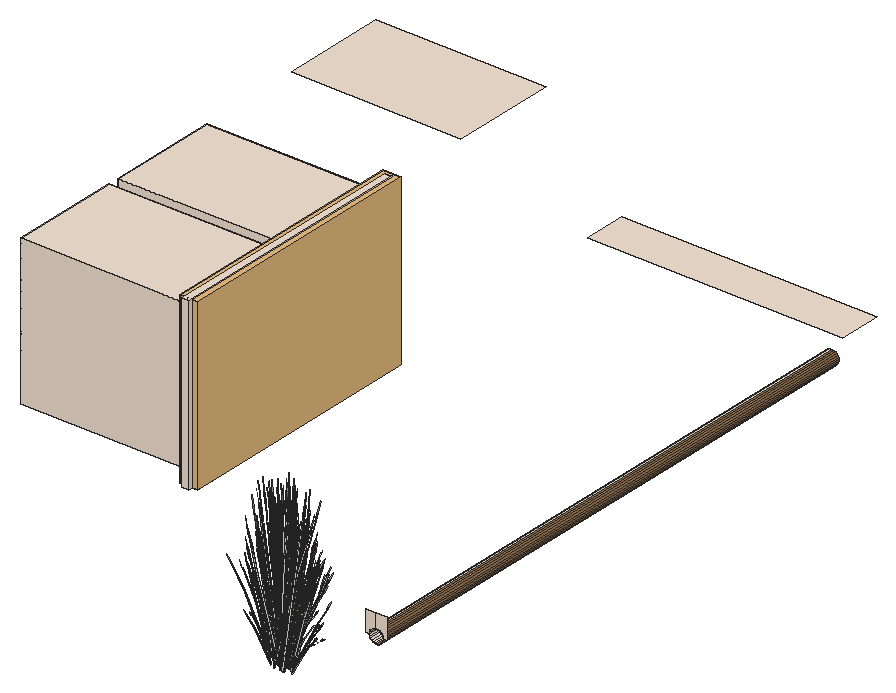
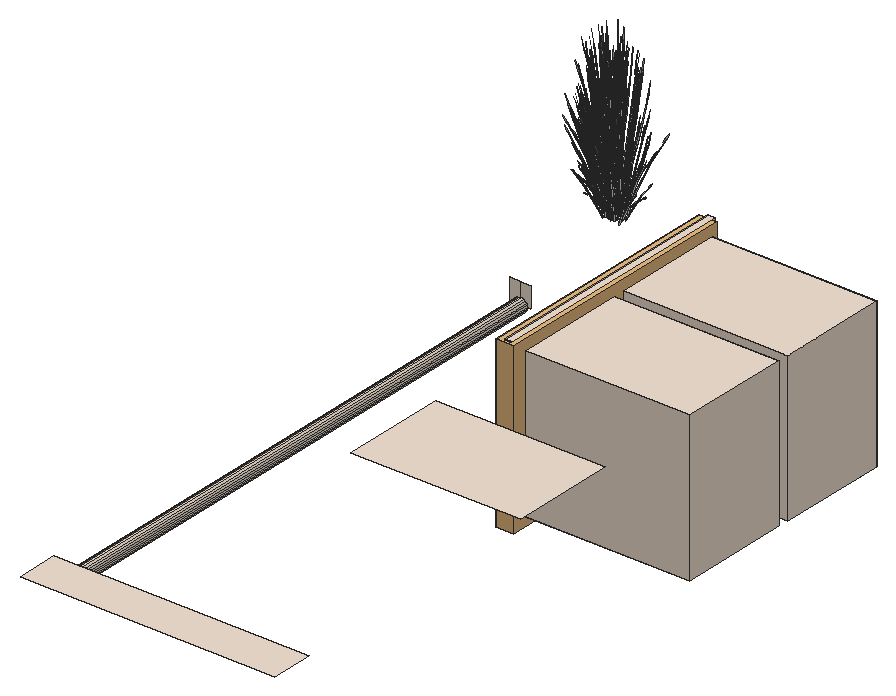
# SketchUp Ruby script. Lengths in inches.
U = 1.inch
M = Sketchup.active_model
def pt(a) = Geom::Point3d.new(a.map { |v| v * U })
def face(e, loops, mat)
  f = e.add_face(loops[0].map { |a| pt(a) })
  loops[1..].each { |l| e.add_face(l.map { |a| pt(a) }).erase! }
  f.material = f.back_material = mat if mat
  f
end
# faces: each face lists its corners as indices into pts; further lists are holes
def faces(e, pts, list, mat = nil) = list.each { |f| face(e, (f[0].is_a?(Array) ? f : [f]).map { |l| l.map { |i| pts[i] } }, mat) }
# xy, xz, yz: faces in a plane at the given z, y or x. An outline is a flat list of corners, or four numbers for a rectangle; further outlines are holes
def ring(l) = l.size == 4 ? [[l[0], l[1]], [l[2], l[1]], [l[2], l[3]], [l[0], l[3]]] : l.each_slice(2).to_a
def flat(e, list, mat, &to3) = list.each { |f| face(e, (f[0].is_a?(Array) ? f : [f]).map { |l| ring(l).map { |u, v| to3.(u, v) } }, mat) }
def xy(e, z, list, mat = nil) = flat(e, list, mat) { |x, y| [x, y, z] }
def xz(e, y, list, mat = nil) = flat(e, list, mat) { |x, z| [x, y, z] }
def yz(e, x, list, mat = nil) = flat(e, list, mat) { |y, z| [x, y, z] }
def lines(e, pts, list) = list.each { |a, b| e.add_line(pt(pts[a]), pt(pts[b])) }
# prism: a flat outline (further loops are holes) pulled along v
def prism(e, loops, v, mat = nil)
  f = face(e, loops, mat); d = Geom::Vector3d.new(v.map { |x| x * U })
  f.pushpull(f.normal.samedirection?(d) ? d.length : -d.length)
end
def box(e, o, s, mat = nil) = prism(e, [[o, [o[0] + s[0], o[1], o[2]], [o[0] + s[0], o[1] + s[1], o[2]], [o[0], o[1] + s[1], o[2]]]], [0, 0, s[2]], mat)
def at(x, y, z, deg = 0) = Geom::Transformation.translation(pt([x, y, z])) * Geom::Transformation.rotation(ORIGIN, Z_AXIS, deg.degrees)
def axes(o, x, y, z) = Geom::Transformation.new([*x, 0, *y, 0, *z, 0, *pt(o).to_a, 1])
def part(name) = M.definitions.add(name)
# library, detail: a bought-in or finely detailed component or shape, given as its bounding box
def library(name, o, s) = part(name).tap { |d| box(d.entities, o, s) }
def detail(e, o, s) = box(e.add_group.entities, o, s)
def put(e, d, t, mat = nil) = e.add_instance(d, t).tap { |i| i.material = mat if mat }
def group(e, t, mat = nil) = e.add_group.tap { |g| g.transformation = t; g.material = mat if mat }.entities
root = M.entities
M.materials.add("C01_Vanilla_Cream").color = [244, 228, 212]
M.materials.add("LightPink_Translucent").color = [144, 107, 117]
M.materials["LightPink_Translucent"].alpha = 0.75
M.materials.add("Wood_Floor_01_1K").color = [146, 111, 76]
c1 = part("blade")
p = [[2.15,0.21,22],[0,0.17,0],[0.09,0.45,0],[2.18,0.31,22],[2.29,0.31,22],[0.38,0.45,0],
  [2.48,0.24,33],[2.49,0.24,33],[2.48,0.22,33]]
faces(c1.entities,p,[[0,1,2,3],[4,5,2,3],[6,3,4,7],[8,0,3,6]])
c2 = part("seeds")
p = [[0.3,-0.1,1.38],[-0.01,-0.03,1.59],[-0.01,-0.03,0.03],[0.14,-0.07,-0.07],[0.29,-0.03,3],[0.15,0.01,3.11]]
faces(c2.entities,p,[[0,1,2,3],[1,0,4,5]],"LightPink_Translucent")
c3 = part("blade with seeds")
put(c3.entities,c1,at(0,0,0))
put(c3.entities,c2,axes([2.4,0.25,30.99],[1.5799,-0.05474,1.17369],[-0.12525,1.92788,0.29478],[-0.07173,-0.02425,1.56792]))
c4 = library("Double casement window",[0,0,0],[5.02,56.42,60])
xy(root,198,[[288,324,290,396],[288,468,360,480]],"C01_Vanilla_Cream")
xy(root,201,[[240,327,290,358.5],[240,361.5,290,393]],"C01_Vanilla_Cream")
xy(root,243,[[240,327,290,358.5],[240,361.5,290,393],[240,423,288,453]],"C01_Vanilla_Cream")
xy(root,246,[[288,324,290,396]],"C01_Vanilla_Cream")
xz(root,306.76,[[354,192,354,198,357,198,357,194,356.48,193.93,356,193.73,355.59,193.41,355.27,193,355.07,192.52,355,192],[359,192,358.93,192.52,358.73,193,358.41,193.41,358,193.73,357.52,193.93,357,194,357,198,360,198,360,192]],"C01_Vanilla_Cream")
xz(root,324,[[288,198,290,246]],"C01_Vanilla_Cream")
xz(root,327,[[240,201,290,243]],"C01_Vanilla_Cream")
xz(root,358.5,[[240,201,290,243]],"C01_Vanilla_Cream")
xz(root,361.5,[[240,201,290,243]],"C01_Vanilla_Cream")
xz(root,393,[[240,201,290,243]],"C01_Vanilla_Cream")
xz(root,396,[[288,198,290,246]],"C01_Vanilla_Cream")
yz(root,240,[[327,201,358.5,243],[361.5,201,393,243]],"C01_Vanilla_Cream")
yz(root,290,[[[324,198,396,246],[327,201,358.5,243],[361.5,201,393,243]]],"C01_Vanilla_Cream")
p = [[357,306.76,190],[356.48,306.76,190.07],[356.48,468,190.07],[357,468,190],[357.52,306.76,190.07],[357.52,468,190.07],
  [356,306.76,190.27],[356,468,190.27],[358,306.76,190.27],[358,468,190.27],[355.59,306.76,190.59],[355.59,468,190.59],
  [358.41,306.76,190.59],[358.41,468,190.59],[355.27,306.76,191],[355.27,468,191],[358.73,306.76,191],[358.73,468,191],
  [355.07,306.76,191.48],[355.07,468,191.48],[358.93,306.76,191.48],[358.93,468,191.48],[355,306.76,192],[355,468,192],
  [359,306.76,192],[359,468,192],[355.07,306.76,192.52],[355.07,468,192.52],[358.93,306.76,192.52],[358.93,468,192.52],
  [355.27,306.76,193],[355.27,468,193],[358.73,306.76,193],[358.73,468,193],[355.59,306.76,193.41],[355.59,468,193.41],
  [358.41,306.76,193.41],[358.41,468,193.41],[356,306.76,193.73],[356,468,193.73],[358,306.76,193.73],[358,468,193.73],
  [356.48,306.76,193.93],[356.48,468,193.93],[357.52,306.76,193.93],[357.52,468,193.93],[357,306.76,194],[357,468,194]]
faces(root,p,[[0,1,2,3],[1,6,7,2],[6,10,11,7],[10,14,15,11],[14,18,19,15],[18,22,23,19],[22,26,27,23],[26,30,31,27],
  [30,34,35,31],[34,38,39,35],[38,42,43,39],[42,46,47,43]],"C01_Vanilla_Cream")
faces(root,p,[[4,0,3,5],[8,4,5,9],[12,8,9,13],[16,12,13,17],[20,16,17,21],[24,20,21,25],[28,24,25,29],[32,28,29,33],
  [36,32,33,37],[40,36,37,41],[44,40,41,45],[46,44,45,47]],"Wood_Floor_01_1K")
put(root,c3,axes([359.88,272.5,201.51],[0.15083,-0.44814,-0.38324],[0.51712,0.15361,-0.29685],[0.2082,-0.04109,0.7333]))
put(root,c3,axes([359.0625,270.67,199.78],[0.34808,-0.49367,0],[0.58235,0.27531,-0.38706],[0.13264,0.0627,1.22783]))
put(root,c3,axes([354.96,271.65,200.91],[0.23093,-0.01116,1.28532],[-0.15319,0.4836,0.10393],[-0.32909,-0.02991,0.54946]))
put(root,c3,axes([356.98,272.78,199.66],[-0.33445,-0.41351,-0.33554],[0.50659,-0.29119,0.16149],[-0.10823,-0.05117,1.07733]))
put(root,c3,axes([357.05,272.2,199.77],[0.24206,0.5509,0.34316],[-0.69162,0.19157,0.13466],[0.00845,-0.10123,1.19142]))
put(root,c3,axes([360.43,272.625,199.49],[-0.35858,0.05912,1.06187],[-0.05708,-0.47061,0.06078],[0.25115,-0.07123,0.60425]))
put(root,c3,axes([361.08,272.21,199.7],[-0.34516,-0.31503,-0.04866],[0.37803,-0.28865,-0.22062],[0.10711,-0.02032,0.72768]))
put(root,c3,axes([356.92,272.63,200.04],[-0.27012,0.44393,0.33554],[-0.56127,-0.21365,-0.16149],[0,-0.10233,1.07733]))
put(root,c3,axes([357.92,272.25,199.65],[0,-0.57005,0],[0.69617,0,0],[0,0,1.34592]))
put(root,c3,axes([358.76,270.93,199.86],[-0.52105,-0.24633,0.37238],[0.31144,-0.44171,0],[0.11867,0.0561,1.18128]))
put(root,c3,axes([359.78,272.66,201.74],[0.48922,-0.21758,-0.53284],[0.27264,0.44789,0.0643],[0.23638,-0.05088,0.75375]))
put(root,c3,axes([356.68,272.94,199.54],[-0.57914,-0.08077,-0.46765],[0.12221,-0.49823,-0.12274],[-0.17283,-0.06037,1.03225]))
put(root,c3,axes([357.59,271.89,199.77],[-0.46162,0.4471,0.34316],[-0.54842,-0.39467,0.13466],[0.11129,-0.04462,1.19142]))
put(root,c3,axes([358.09,272.6875,199.72],[-0.51786,-0.42404,-0.04598],[0.51817,-0.4243,0],[-0.01808,-0.01481,1.31678]))
put(root,c3,axes([356.79,271.15,199.86],[-0.16083,0.48962,0.13232],[-0.58854,-0.13856,0.26315],[0.10167,-0.00238,1.20305]))
put(root,c3,axes([359.71,272.75,201.79],[-0.46269,-0.13744,0.2656],[0.13495,-0.40096,-0.3429],[0.18628,-0.03677,0.65611]))
put(root,c3,axes([354.86,272.01,201.55],[0.15729,-0.44921,0.36002],[0.51712,0.15361,0.29685],[-0.20336,0.027,0.74497]))
put(root,c3,axes([356.54,271.55,199.2],[-0.548,0.19724,0.96696],[-0.17442,-0.56594,0.37572],[0.3365,0.00941,1.09981]))
put(root,c3,axes([358.01,271.7,199.96],[0.1074,-0.43968,0.1086],[0.52474,0.07632,-0.3101],[0.0955,0.04515,0.95058]))
put(root,c3,axes([354.83,271.89,201.55],[-0.20448,-0.33592,0.04823],[0.37288,-0.16442,0.37966],[-0.16437,0.03244,0.57892]))
put(root,c3,axes([357.11,272.74,199.77],[0.70367,0.1038,0.34316],[-0.1432,0.58624,0.13466],[-0.10283,-0.05661,1.19142]))
put(root,c3,axes([360.82,272.32,199.12],[-0.0291,-0.0748,1.32257],[0.20181,-0.43752,-0.20205],[0.20357,-0.00629,0.22528]))
put(root,c3,axes([354.81,272.24,199.12],[0.01412,0.07764,1.32257],[-0.28464,0.40547,-0.20205],[-0.20218,-0.02044,0.22528]))
put(root,c3,axes([357.79,271.8125,200.04],[-0.33445,-0.41351,0.33554],[0.50659,-0.29119,-0.16149],[0.10823,0.05117,1.07733]))
put(root,c3,axes([356.0625,273.7,199.52],[-0.13078,-0.42928,-0.23233],[0.51941,-0.1219,0.23233],[-0.10471,-0.0495,1.0423]))
put(root,c3,axes([356.73,273.68,199.86],[0.59825,-0.13076,0.13232],[0.14773,0.48663,0.26315],[-0.05336,-0.0709,1.20305]))
put(root,c3,axes([357.96,271.84,200],[0.56211,-0.32708,-0.21822],[0.3738,0.46216,-0.37502],[0.13869,0.04694,1.19781]))
put(root,c3,axes([360.2,272.7,201.39],[0.46269,0.13744,-0.2656],[-0.13495,0.40096,0.3429],[0.18628,-0.03677,0.65611]))
put(root,c3,axes([355.92,273.89,199.51],[-0.52105,-0.24633,-0.37238],[0.31144,-0.44171,0],[-0.11867,-0.0561,1.18128]))
put(root,c3,axes([359.38,270.97,199.51],[0.52105,0.24633,-0.37238],[-0.31144,0.44171,0],[0.11867,0.0561,1.18128]))
put(root,c3,axes([354.76,272.0625,201.39],[-0.46269,-0.13744,-0.2656],[0.13495,-0.40096,0.3429],[-0.18628,0.03677,0.65611]))
put(root,c3,axes([358.39,272.375,199.65],[0.62289,0,0],[0,0.51004,0],[0,0,1.33805]))
put(root,c3,axes([357.33,273.02,200],[-0.56211,0.32708,-0.21822],[-0.3738,-0.46216,-0.37502],[-0.13869,-0.04694,1.19781]))
put(root,c3,axes([358.57,271.18,199.86],[-0.59825,0.13076,0.13232],[-0.14773,-0.48663,0.26315],[0.05336,0.0709,1.20305]))
put(root,c3,axes([358.93,272.21,200.91],[-0.23093,0.01116,1.28532],[0.15319,-0.4836,0.10393],[0.32909,0.02991,0.54946]))
put(root,c3,axes([359.23,271.15,199.52],[0.13078,0.42928,-0.23233],[-0.51941,0.1219,0.23233],[0.10471,0.0495,1.0423]))
put(root,c3,axes([360.13,272.87,201.55],[0.20448,0.33592,0.04823],[-0.37288,0.16442,0.37966],[0.16437,-0.03244,0.57892]))
put(root,c3,axes([358.1875,272.12,199.79],[-0.70367,-0.1038,0.36899],[0.1432,-0.58624,0.1448],[0.10283,0.05661,1.2811]))
put(root,c3,axes([360.09,272.75,201.55],[-0.15729,0.44921,0.36002],[-0.51712,-0.15361,0.29685],[0.20336,-0.027,0.74497]))
put(root,c3,axes([357.625,273.5625,199.65],[-0.18165,-0.42474,0],[0.51872,-0.14874,0],[0,0,1.15778]))
put(root,c3,axes([357.28,273.16,199.96],[-0.1074,0.43968,0.1086],[-0.52474,-0.07632,-0.3101],[-0.0955,-0.04515,0.95058]))
put(root,c3,axes([355.24,272.02,201.79],[0.46269,0.13744,0.2656],[-0.13495,0.40096,-0.3429],[-0.18628,0.03677,0.65611]))
put(root,c3,axes([358.31,273.5,199.64],[0.5845,-0.16716,-0.14398],[0.20539,0.48152,0.00006],[0.06452,-0.01848,1.30423]))
put(root,c3,axes([358.51,273.7,199.86],[0.16083,-0.48962,0.13232],[0.58854,0.13856,0.26315],[-0.10167,0.00238,1.20305]))
put(root,c3,axes([358.375,272.59,199.66],[0.38863,0.31822,0],[-0.38863,0.31822,0],[0,0,1.2695]))
put(root,c3,axes([356.17,272,200.51],[0.15825,-0.07127,1.32798],[0.05457,0.4976,0.10393],[-0.34278,0.06603,0.47463]))
put(root,c3,axes([359.43,272.45,199.86],[-0.43742,-0.35886,0.13232],[0.44081,-0.34807,0.26315],[-0.04831,0.07329,1.20305]))
put(root,c3,axes([358.62,271.91,199.54],[0.57914,0.08077,-0.46765],[-0.12221,0.49823,-0.12274],[0.17283,0.06037,1.03225]))
put(root,c3,axes([361.18,272.78,200.07],[-0.34399,0.08133,0.86145],[0.16192,-0.33614,0.63294],[0.18249,0.023,0.18974]))
put(root,c3,axes([357.5,273.75,199.65],[-0.56127,-0.22118,0],[0.27012,-0.45959,0],[0,0,1.2203]))
put(root,c3,axes([357.96,273.17,199.85],[-0.54364,-0.39653,-0.18894],[0.45745,-0.44527,0.41347],[-0.14639,0.04639,1.26162]))
put(root,c3,axes([356.53,273.93,199.86],[0.52105,0.24633,0.37238],[-0.31144,0.44171,0],[-0.11867,-0.0561,1.18128]))
put(root,c3,axes([358.37,272.22,200.04],[0.27012,-0.44393,0.33554],[0.56127,0.21365,-0.16149],[0,0.10233,1.07733]))
put(root,c3,axes([361.02,274.21,201.53],[-0.05034,-0.04313,1.33037],[0.11012,-0.46232,-0.12571],[0.1983,-0.02954,0.23543]))
put(root,c3,axes([354.47,272.33,201.54],[-0.09091,0.06396,1.31208],[0.00773,0.46734,-0.2075],[-0.20839,0.06078,0.10523]))
put(root,c3,axes([358.27,272.48,199.72],[0,0.56976,-0.04228],[-0.69617,0,0],[0,0.01791,1.34526]))
put(root,c3,axes([355.07,272.27,201.51],[-0.15083,0.44814,-0.38324],[-0.51712,-0.15361,-0.29685],[-0.2082,0.04109,0.7333]))
put(root,c3,axes([355.05,271.88,201.78],[0.28012,0.44611,-0.0912],[-0.49717,0.21923,-0.50621],[-0.20951,0.05886,0.76918]))
put(root,c3,axes([358.32,272.07,199.66],[0.33445,0.41351,-0.33554],[-0.50659,0.29119,0.16149],[0.10823,0.05117,1.07733]))
put(root,c3,axes([360.58,273.82,200.95],[-0.10656,-0.41414,-0.02619],[0.50364,-0.09521,-0.11874],[0.10517,0.02626,0.39164]))
put(root,c3,axes([356.23,274.18,199.78],[-0.34808,0.49367,0],[-0.58235,-0.27531,-0.38706],[-0.13264,-0.0627,1.22783]))
put(root,c3,axes([359.27,273.81,201.78],[0.02981,-0.50103,-0.0912],[0.56442,0.01369,-0.50621],[0.21738,0.0348,0.76918]))
put(root,c3,axes([359.79,272.47,199.86],[0,-0.49266,0.37238],[0.62289,0,0],[0,0.11221,1.18128]))
put(root,c3,axes([358.23,272.84,200.04],[0.60457,-0.03041,0.33554],[0.05467,0.50484,-0.16149],[-0.10823,0.05117,1.07733]))
put(root,c3,axes([358.6,272.32,199.96],[0.51872,-0.14368,0.1086],[0.18165,0.41027,-0.3101],[0,0.09029,0.95058]))
put(root,c3,axes([359.1875,273.61,201.79],[-0.31678,-0.30846,0.2656],[0.36171,-0.29199,-0.3429],[0.18378,0.04443,0.65611]))
put(root,c3,axes([357.6875,273.08,199.66],[-0.60457,0.03041,-0.33554],[-0.05467,-0.50484,0.16149],[-0.10823,0.05117,1.07733]))
put(root,c3,axes([360.53,273.32,199.94],[-0.13408,-0.12117,1.07251],[0.17446,-0.40083,-0.23066],[0.27128,0.0543,0.45856]))
put(root,c3,axes([358.14,273.76,199.65],[0.56127,0.22118,0],[-0.27012,0.45959,0],[0,0,1.31215]))
put(root,c3,axes([359.76,273.51,201.54],[0.11943,-0.00833,1.31208],[0.32759,-0.38275,-0.2075],[0.21244,0.05052,0.10523]))
put(root,c3,axes([358.36,274.25,199.64],[-0.34375,-0.4954,-0.03857],[0.58235,-0.27531,0.38706],[-0.1435,0.04717,1.22723]))
put(root,c3,axes([358.24,273.05,199.96],[0.41131,0.296,0.1086],[-0.34309,0.33395,-0.3101],[-0.0955,0.04515,0.95058]))
put(root,c3,axes([354.99,273.13,201.55],[-0.13808,-0.45342,0.36002],[0.54163,-0.07869,0.29685],[-0.15963,0.10664,0.74497]))
put(root,c3,axes([354.88,273.04,201.55],[-0.3822,-0.20719,0.04823],[0.22252,-0.29505,0.37966],[-0.12254,0.09539,0.57892]))
put(root,c3,axes([355.06,272.5,200.91],[0.19317,-0.10421,1.28532],[0.16263,0.48153,0.10393],[-0.30326,0.10883,0.54946]))
put(root,c3,axes([359.3,273.57,201.74],[0.55654,0.01186,-0.53284],[-0.03738,0.49951,0.0643],[0.23578,0.05271,0.75375]))
put(root,c3,axes([358.67,273.97,199.86],[0.52105,-0.24633,0.37238],[0.31144,0.44171,0],[-0.11867,0.0561,1.18128]))
put(root,c3,axes([357.93,273.58,199.72],[0.24206,0.56598,-0.04509],[-0.69162,0.19832,0],[0.00845,0.01976,1.2913]))
put(root,c3,axes([358.2,274.19,199.52],[-0.51941,-0.1219,-0.23233],[0.13078,-0.42928,0.23233],[-0.10471,0.0495,1.0423]))
put(root,c3,axes([354.45,273.32,199.94],[0.19348,0.04044,1.07251],[0.1247,0.41309,-0.23066],[-0.26282,0.07733,0.45856]))
put(root,c3,axes([355.32,272.98,201.79],[0.48462,-0.07041,0.2656],[0.12797,0.4025,-0.3429],[-0.13888,0.10811,0.65611]))
put(root,c3,axes([360.21,272.55,199.78],[0.69617,0,0],[0,0.55062,-0.38706],[0,0.12541,1.22783]))
put(root,c3,axes([353.46,272.8,201.53],[0.07105,0.01321,1.33037],[0.2198,0.43529,-0.12571],[-0.14545,0.11425,0.23543]))
put(root,c3,axes([359.93,272.84,199.65],[-0.69582,-0.00394,-0.03732],[0,-0.55062,0.37457],[-0.02187,0.12535,1.18764]))
put(root,c3,axes([358.43,272.36,200],[0.62699,0.23507,-0.21822],[-0.3019,0.49615,-0.37502],[0.0197,0.12182,1.19781]))
put(root,c3,axes([354.05,274.18,200.07],[0.23202,-0.22328,0.86145],[0.09155,0.35348,0.63294],[-0.16768,0.06329,0.18974]))
put(root,c3,axes([359.64,273.77,201.39],[0.31678,0.30846,-0.2656],[-0.36171,0.29199,0.3429],[0.18378,0.04443,0.65611]))
put(root,c3,axes([359.79,272.92,199.52],[-0.38863,0.30738,-0.23233],[-0.38863,-0.30738,0.23233],[0,0.09901,1.0423]))
put(root,c3,axes([358.11,272.95,200],[0.06488,0.56215,-0.21822],[-0.6757,0.03399,-0.37502],[-0.11898,0.07488,1.19781]))
put(root,c3,axes([359.47,273.89,201.55],[-0.02803,0.37463,0.04823],[-0.42332,-0.01027,0.37966],[0.16216,0.0392,0.57892]))
put(root,c3,axes([358.36,272.73,199.66],[-0.27012,0.44393,-0.33554],[-0.56127,-0.21365,0.16149],[0,0.10233,1.07733]))
put(root,c3,axes([354.93,273.22,201.39],[-0.48462,0.07041,-0.2656],[-0.12797,-0.4025,0.3429],[-0.13888,0.10811,0.65611]))
put(root,c3,axes([359.51,273.77,201.55],[-0.41051,0.32462,0.36002],[-0.35404,-0.34474,0.29685],[0.1926,0.05988,0.74497]))
put(root,c3,axes([354.22,274.125,202.23],[0.49129,0.13151,-0.04866],[-0.15113,0.40475,-0.22062],[-0.08035,0.06145,0.72768]))
put(root,c3,axes([357.71,273.375,199.54],[-0.375,0.3703,-0.46765],[-0.46584,-0.33578,-0.12274],[-0.15027,0.09237,1.03225]))
put(root,c3,axes([358.21,274.15,201.79],[-0.08599,-0.39682,0.2656],[0.49155,-0.10478,-0.3429],[0.13203,0.11372,0.65611]))
put(root,c3,axes([358.375,274,199.75],[0.697,0.16013,0.23067],[-0.17437,0.57237,-0.27369],[-0.11536,0.07164,1.23664]))
put(root,c3,axes([358.32,274.38,199.51],[-0.52105,0.24633,-0.37238],[-0.31144,-0.44171,0],[-0.11867,0.0561,1.18128]))
put(root,c3,axes([360.06,272.93,199.51],[0,0.49266,-0.37238],[-0.62289,0,0],[0,0.11221,1.18128]))
put(root,c3,axes([358.5,272.98,200.91],[-0.2068,-0.08488,1.28532],[0.42797,-0.35609,0.10393],[0.26673,0.16064,0.54946]))
put(root,c3,axes([358.54,271.86,201.36],[-0.48108,-0.25598,1.03712],[0.50798,-0.39855,0.44749],[0.15521,0.24018,1.00248]))
put(root,c3,axes([355.07,272.94,201.78],[0.515,0.27165,-0.0912],[-0.2967,0.3934,-0.50621],[-0.1455,0.13675,0.76918]))
put(root,c3,axes([359.26,273.95,200.07],[-0.31347,-0.14166,0.86145],[0.40476,-0.14393,0.63294],[0.10917,0.12192,0.18974]))
put(root,c3,axes([358.16,274.35,201.78],[0.33176,-0.4217,-0.0912],[0.48044,0.24295,-0.50621],[0.16701,0.11914,0.76918]))
put(root,c3,axes([355.76,272.82,200.91],[0.13906,-0.15138,1.28532],[0.35111,0.40859,0.10393],[-0.24082,0.18608,0.54946]))
put(root,c3,axes([355.33,273.27,201.51],[0.14302,0.44985,-0.38324],[-0.54163,0.07869,-0.29685],[-0.15522,0.12083,0.7333]))
put(root,c3,axes([355.98,273.78,201.79],[0.3767,-0.25939,0.2656],[0.3566,0.29618,-0.3429],[-0.05426,0.15048,0.65611]))
put(root,c3,axes([358.8,274.31,199.78],[0.34808,0.49367,0],[-0.58235,0.27531,-0.38706],[-0.13264,0.0627,1.22783]))
put(root,c3,axes([357.73,274.7,201.53],[0.00165,-0.05965,1.33037],[0.47711,-0.26315,-0.12571],[0.16572,0.09393,0.23543]))
put(root,c3,axes([359.35,274.47,199.12],[0.04056,-0.07113,1.32257],[0.51066,-0.20948,-0.20205],[0.15482,0.10842,0.22528]))
put(root,c3,axes([358.5,272.35,200.13],[-0.01521,-0.46386,1.05954],[0.68831,0.12024,0.44862],[-0.1628,0.25382,1.00012]))
put(root,c3,axes([358.68,272.86,199.57],[0.20414,0.45107,-0.51909],[-0.58805,0.16245,-0.13624],[0.02256,0.15274,1.1458]))
put(root,c3,axes([355.63,274.02,201.55],[-0.45752,-0.02296,0.04823],[0.01254,-0.34663,0.37966],[-0.04787,0.13278,0.57892]))
put(root,c3,axes([354.66,274.41,199.12],[0.07468,0.04922,1.32257],[0.12663,0.45605,-0.20205],[-0.16551,0.09725,0.22528]))
put(root,c3,axes([355.78,274.05,201.55],[-0.39645,-0.33614,0.36002],[0.42102,-0.2899,0.29685],[-0.07313,0.15771,0.74497]))
put(root,c3,axes([358.56,274.14,201.51],[0.54938,-0.11711,-0.38324],[0.0961,0.44351,-0.29685],[0.14756,0.1271,0.7333]))
put(root,c3,axes([357.03,274.21,201.79],[0.16784,-0.37886,0.2656],[0.48968,0.1105,-0.3429],[0.0449,0.15254,0.65611]))
put(root,c3,axes([359.3125,274.59,200],[-0.35702,-0.01545,0.78795],[0.23577,-0.32816,0.43504],[0.14104,0.11659,0.61808]))
put(root,c3,axes([358.29,274.51,201.55],[-0.25304,0.31296,0.04823],[-0.36033,-0.18221,0.37966],[0.11649,0.10034,0.57892]))
put(root,c3,axes([357.69,275.5625,202.23],[0.38473,-0.28263,-0.04866],[0.35252,0.30954,-0.22062],[0.02482,0.08771,0.72768]))
put(root,c3,axes([358.39,274.42,201.55],[-0.55374,0.11306,0.36002],[-0.0961,-0.44351,0.29685],[0.13023,0.13071,0.74497]))
put(root,c3,axes([355.66,273.2,200.91],[0.10366,-0.16934,1.28532],[0.43488,0.35044,0.10393],[-0.19618,0.21841,0.54946]))
put(root,c3,axes([358.15,273.8,199.94],[0.00982,-0.16331,1.07251],[0.4695,-0.18242,-0.23066],[0.14493,0.19547,0.45856]))
put(root,c3,axes([356.88,274.55,201.55],[-0.41024,0.16744,0.04823],[-0.2008,-0.30532,0.37966],[0.03962,0.13459,0.57892]))
put(root,c3,axes([355.78,274.15,201.39],[-0.3767,0.25939,-0.2656],[-0.3566,-0.29618,0.3429],[-0.05426,0.15048,0.65611]))
put(root,c3,axes([354.48,274.07,201.54],[-0.01384,0.09749,1.31208],[0.39274,0.33916,-0.2075],[-0.10282,0.16039,0.10523]))
put(root,c3,axes([355.74,273.85,202.05],[0.61188,0.02441,-0.10123],[-0.01672,0.46217,-0.56189],[-0.0425,0.178,0.85379]))
put(root,c3,axes([356.87,274.37,201.78],[0.54481,-0.22937,-0.0912],[0.26773,0.4071,-0.50621],[0.07188,0.17155,0.76918]))
put(root,c3,axes([357.03,274.52,201.8],[-0.54859,-0.1288,0.39962],[0.18759,-0.42344,0.32951],[0.03297,0.16652,0.82692]))
put(root,c3,axes([356.02,275.16,200.07],[-0.01441,-0.29294,0.86145],[0.36003,0.20894,0.63294],[-0.07081,0.13963,0.18974]))
put(root,c3,axes([356.97,274.46,199.12],[0.0901,-0.02681,1.32257],[0.54199,0.14755,-0.20205],[0.01585,0.1663,0.22528]))
put(root,c3,axes([356.15,274.03,201.75],[0.39855,0.33102,-0.4254],[-0.42102,0.2899,-0.32951],[-0.06064,0.16819,0.81396]))
put(root,c3,axes([355.72,274.53,200.12],[0.50577,-0.08724,0.04881],[0.11627,0.35148,-0.64728],[-0.03206,0.17792,0.5802]))
put(root,c3,axes([357.34,274.35,201.51],[0.54728,0.1235,-0.38324],[-0.18759,0.42344,-0.29685],[0.05018,0.17048,0.7333]))
put(root,c3,axes([357.65,273.48,200.91],[-0.12726,-0.15818,1.28532],[0.58807,-0.13317,0.10393],[0.13291,0.24832,0.54946]))
put(root,c3,axes([357.09,274.61,201.39],[-0.16784,0.37886,-0.2656],[-0.48968,-0.1105,0.3429],[0.0449,0.15254,0.65611]))
put(root,c3,axes([356.03,273.875,202],[-0.01449,0.45571,-0.59145],[-0.61002,-0.03061,0.07138],[-0.06438,0.19306,0.83667]))
put(root,c3,axes([354.4375,275.07,201.53],[0.06316,-0.02974,1.33037],[0.52204,0.19785,-0.12571],[-0.01227,0.16473,0.23543]))
put(root,c3,axes([356.61,273.55,200.91],[-0.01363,-0.18909,1.28532],[0.5906,0.12544,0.10393],[-0.03653,0.26947,0.54946]))
put(root,c3,axes([357.14,274.27,201.74],[0.26572,0.40059,-0.53284],[-0.54698,0.22325,0.0643],[0.06214,0.19355,0.75375]))
put(root,c3,axes([355.6,274.9,199.94],[0.17569,-0.07772,1.07251],[0.43377,0.23434,-0.23066],[-0.12911,0.20277,0.45856]))
put(root,c3,axes([356.74,275.28,201.54],[0.07057,0.07933,1.31208],[0.56952,0.03117,-0.2075],[0.05727,0.17496,0.10523]))
put(root,c3,axes([355.83,274.52,200.52],[0.01223,-0.25433,1.15759],[0.55017,0.13434,0.15997],[-0.04767,0.27105,0.54661]))
put(root,c4,axes([286.7,325.0625,198.3],[1,0,0],[0,1.27666,0],[0,0,0.79394]))
